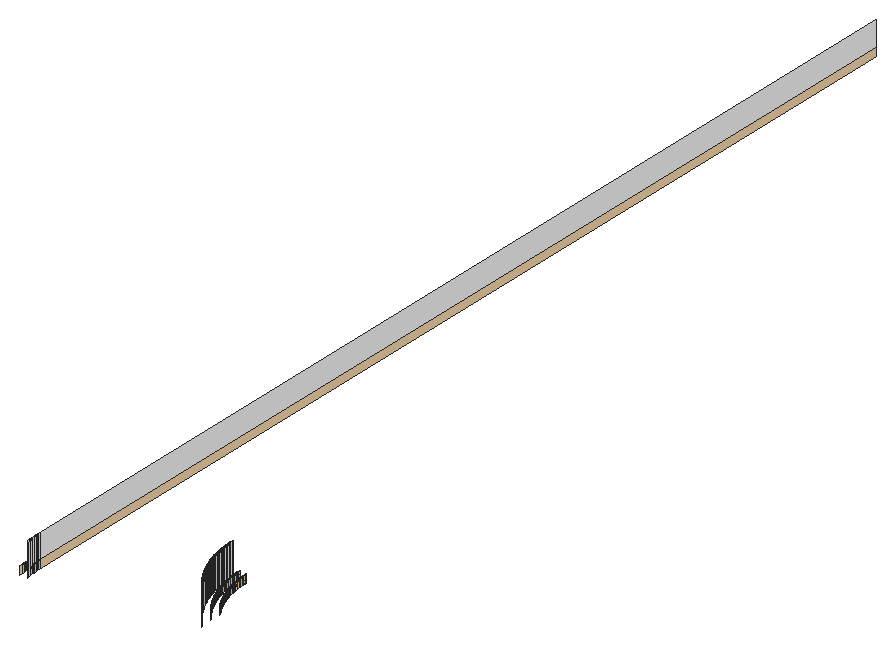
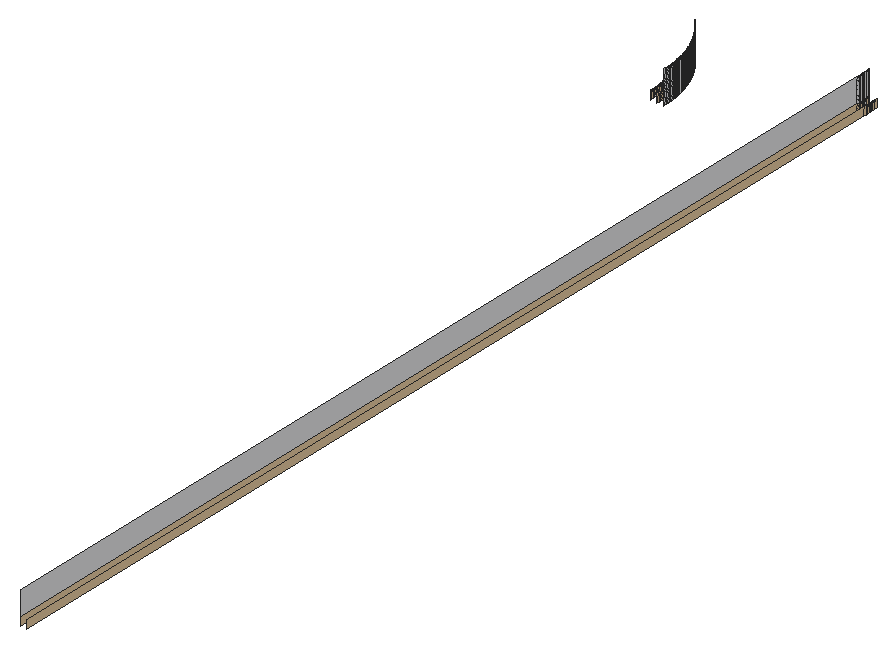
# SketchUp Ruby script. Lengths in inches.
U = 1.inch
M = Sketchup.active_model
def pt(a) = Geom::Point3d.new(a.map { |v| v * U })
def face(e, loops, mat)
  f = e.add_face(loops[0].map { |a| pt(a) })
  loops[1..].each { |l| e.add_face(l.map { |a| pt(a) }).erase! }
  f.material = f.back_material = mat if mat
  f
end
# faces: each face lists its corners as indices into pts; further lists are holes
def faces(e, pts, list, mat = nil) = list.each { |f| face(e, (f[0].is_a?(Array) ? f : [f]).map { |l| l.map { |i| pts[i] } }, mat) }
# xy, xz, yz: faces in a plane at the given z, y or x. An outline is a flat list of corners, or four numbers for a rectangle; further outlines are holes
def ring(l) = l.size == 4 ? [[l[0], l[1]], [l[2], l[1]], [l[2], l[3]], [l[0], l[3]]] : l.each_slice(2).to_a
def flat(e, list, mat, &to3) = list.each { |f| face(e, (f[0].is_a?(Array) ? f : [f]).map { |l| ring(l).map { |u, v| to3.(u, v) } }, mat) }
def xy(e, z, list, mat = nil) = flat(e, list, mat) { |x, y| [x, y, z] }
def xz(e, y, list, mat = nil) = flat(e, list, mat) { |x, z| [x, y, z] }
def yz(e, x, list, mat = nil) = flat(e, list, mat) { |y, z| [x, y, z] }
def lines(e, pts, list) = list.each { |a, b| e.add_line(pt(pts[a]), pt(pts[b])) }
# prism: a flat outline (further loops are holes) pulled along v
def prism(e, loops, v, mat = nil)
  f = face(e, loops, mat); d = Geom::Vector3d.new(v.map { |x| x * U })
  f.pushpull(f.normal.samedirection?(d) ? d.length : -d.length)
end
def box(e, o, s, mat = nil) = prism(e, [[o, [o[0] + s[0], o[1], o[2]], [o[0] + s[0], o[1] + s[1], o[2]], [o[0], o[1] + s[1], o[2]]]], [0, 0, s[2]], mat)
def at(x, y, z, deg = 0) = Geom::Transformation.translation(pt([x, y, z])) * Geom::Transformation.rotation(ORIGIN, Z_AXIS, deg.degrees)
def axes(o, x, y, z) = Geom::Transformation.new([*x, 0, *y, 0, *z, 0, *pt(o).to_a, 1])
def part(name) = M.definitions.add(name)
# library, detail: a bought-in or finely detailed component or shape, given as its bounding box
def library(name, o, s) = part(name).tap { |d| box(d.entities, o, s) }
def detail(e, o, s) = box(e.add_group.entities, o, s)
def put(e, d, t, mat = nil) = e.add_instance(d, t).tap { |i| i.material = mat if mat }
def group(e, t, mat = nil) = e.add_group.tap { |g| g.transformation = t; g.material = mat if mat }.entities
root = M.entities
M.materials.add("False Ceiling Light").color = [254, 223, 179]
M.materials.add("[Quartz Light Grey]").color = [251, 251, 252]
yz(root,22.5,[[65.53,115.32,65.76,116.49],[65.76,115.32,66,116.49],[66,115.32,216,116.49]],"False Ceiling Light")
yz(root,23.5,[[65.55,115.32,65.77,116.49],[65.77,115.32,66.01,116.49],[66.01,115.32,215.99,116.49]],"False Ceiling Light")
yz(root,23.5,[[65.55,115.32,65.77,120],[65.77,115.32,66.01,120],[66.01,115.32,215.99,120]],"[Quartz Light Grey]")
yz(root,41.5,[[77.67,115.32,77.88,120],[77.88,115.32,78.06,120]],"[Quartz Light Grey]")
yz(root,42.5,[[77.7,115.32,77.89,116.49],[77.89,115.32,78.0625,116.49]],"False Ceiling Light")
yz(root,43.5,[[77.72,115.32,77.89,116.49],[77.89,115.32,78.0625,116.49]],"False Ceiling Light")
yz(root,43.5,[[77.72,115.32,77.89,115.91],[77.89,115.32,78.0625,115.91]],"[Quartz Light Grey]")
yz(root,43.51,[[77.36,115.32,77.54,116.49]],"False Ceiling Light")
yz(root,43.51,[[77.36,115.32,77.54,115.91]],"[Quartz Light Grey]")
p = [[22.6,63.88,115.32],[22.625,63.65,115.32],[22.625,63.65,116.49],[22.6,63.88,116.49],[23.6,63.98,115.32],[23.62,63.75,115.32],
  [23.62,63.75,120],[23.6,63.98,120],[23.62,63.75,115.32],[23.6,63.98,115.32],[23.6,63.98,116.49],[23.62,63.75,116.49],
  [22.58,64.12,115.32],[22.58,64.12,116.49],[23.58,64.2,115.32],[23.58,64.2,120],[23.58,64.2,115.32],[23.58,64.2,116.49],
  [22.56,64.35,115.32],[22.56,64.35,116.49],[23.56,64.43,115.32],[23.56,64.43,120],[23.56,64.43,115.32],[23.56,64.43,116.49],
  [22.54,64.59,115.32],[22.54,64.59,116.49],[23.54,64.65,115.32],[23.54,64.65,120],[23.54,64.65,115.32],[23.54,64.65,116.49],
  [22.53,64.82,115.32],[22.53,64.82,116.49],[23.53,64.875,115.32],[23.53,64.875,120],[23.53,64.875,115.32],[23.53,64.875,116.49],
  [22.52,65.06,115.32],[22.52,65.06,116.49],[23.52,65.1,115.32],[23.52,65.1,120],[23.52,65.1,115.32],[23.52,65.1,116.49],
  [22.51,65.29,115.32],[22.51,65.29,116.49],[23.51,65.32,115.32],[23.51,65.32,120],[23.51,65.32,115.32],[23.51,65.32,116.49],
  [22.5,65.53,115.32],[22.5,65.53,116.49],[23.5,65.55,115.32],[23.5,65.55,120],[23.5,65.55,115.32],[23.5,65.55,116.49],
  [45.87,67.21,115.32],[45.73,67.36,115.32],[45.73,67.36,120],[45.87,67.21,120],[45.59,67.51,115.32],[45.59,67.51,120],
  [45.45,67.66,115.32],[45.45,67.66,120],[45.32,67.8125,115.32],[45.32,67.8125,120],[45.18,67.97,115.32],[45.18,67.97,120],
  [45.05,68.125,115.32],[45.05,68.125,120],[44.93,68.28,115.32],[44.93,68.28,120],[44.8,68.44,115.32],[44.8,68.44,120],
  [44.67,68.6,115.32],[44.67,68.6,120],[44.55,68.76,115.32],[44.55,68.76,120],[44.43,68.93,115.32],[44.43,68.93,120],
  [45.7,68.91,115.32],[45.82,68.76,115.32],[45.82,68.76,116.49],[45.7,68.91,116.49],[44.3125,69.09,115.32],[44.3125,69.09,120],
  [45.59,69.06,115.32],[45.59,69.06,116.49],[44.2,69.26,115.32],[44.2,69.26,120],[45.47,69.21,115.32],[45.47,69.21,116.49],
  [45.35,69.36,115.32],[45.35,69.36,116.49],[44.08,69.43,115.32],[44.08,69.43,120],[43.97,69.6,115.32],[43.97,69.6,120],
  [45.24,69.51,115.32],[45.24,69.51,116.49],[45.13,69.67,115.32],[45.13,69.67,116.49],[43.86,69.77,115.32],[43.86,69.77,120],
  [45.02,69.83,115.32],[45.02,69.83,116.49],[43.76,69.95,115.32],[43.76,69.95,120],[44.92,69.98,115.32],[44.92,69.98,116.49],
  [43.65,70.12,115.32],[43.65,70.12,120],[44.8125,70.14,115.32],[44.8125,70.14,116.49],[43.55,70.3,115.32],[43.55,70.3,120],
  [44.71,70.3,115.32],[44.71,70.3,116.49],[43.45,70.47,115.32],[43.45,70.47,120],[44.61,70.47,115.32],[44.61,70.47,116.49],
  [43.35,70.65,115.32],[43.35,70.65,120],[44.51,70.63,115.32],[44.51,70.63,116.49],[45.75,70.54,115.32],[45.65,70.68,115.32],
  [45.65,70.68,116.49],[45.75,70.54,116.49],[45.65,70.68,115.32],[45.75,70.54,115.32],[45.75,70.54,115.91],[45.65,70.68,115.91],
  [44.42,70.79,115.32],[44.42,70.79,116.49],[43.26,70.83,115.32],[43.26,70.83,120],[45.56,70.83,115.32],[45.56,70.83,116.49],
  [45.56,70.83,115.32],[45.56,70.83,115.91],[43.16,71.01,115.32],[43.16,71.01,120],[44.32,70.96,115.32],[44.32,70.96,116.49],
  [45.47,70.99,115.32],[45.47,70.99,116.49],[45.47,70.99,115.32],[45.47,70.99,115.91],[43.07,71.2,115.32],[43.07,71.2,120],
  [44.23,71.125,115.32],[44.23,71.125,116.49],[45.375,71.14,115.32],[45.375,71.14,116.49],[45.375,71.14,115.32],[45.375,71.14,115.91],
  [44.14,71.3,115.32],[44.14,71.3,116.49],[45.29,71.29,115.32],[45.29,71.29,116.49],[45.29,71.29,115.32],[45.29,71.29,115.91],
  [42.98,71.38,115.32],[42.98,71.38,120],[44.06,71.46,115.32],[44.06,71.46,116.49],[45.2,71.45,115.32],[45.2,71.45,116.49],
  [45.2,71.45,115.32],[45.2,71.45,115.91],[42.9,71.5625,115.32],[42.9,71.5625,120],[45.11,71.6,115.32],[45.11,71.6,116.49],
  [45.11,71.6,115.32],[45.11,71.6,115.91],[43.97,71.64,115.32],[43.97,71.64,116.49],[42.82,71.75,115.32],[42.82,71.75,120],
  [43.89,71.81,115.32],[43.89,71.81,116.49],[45.03,71.76,115.32],[45.03,71.76,116.49],[45.03,71.76,115.32],[45.03,71.76,115.91],
  [42.73,71.9375,115.32],[42.73,71.9375,120],[43.81,71.98,115.32],[43.81,71.98,116.49],[44.95,71.92,115.32],[44.95,71.92,116.49],
  [44.95,71.92,115.32],[44.95,71.92,115.91],[42.66,72.125,115.32],[42.66,72.125,120],[44.87,72.07,115.32],[44.87,72.07,116.49],
  [44.87,72.07,115.32],[44.87,72.07,115.91],[43.73,72.15,115.32],[43.73,72.15,116.49],[42.58,72.3125,115.32],[42.58,72.3125,120],
  [44.79,72.23,115.32],[44.79,72.23,116.49],[44.79,72.23,115.32],[44.79,72.23,115.91],[43.66,72.33,115.32],[43.66,72.33,116.49],
  [44.72,72.39,115.32],[44.72,72.39,116.49],[44.72,72.39,115.32],[44.72,72.39,115.91],[42.51,72.5,115.32],[42.51,72.5,120],
  [43.58,72.5,115.32],[43.58,72.5,116.49],[44.65,72.56,115.32],[44.65,72.56,116.49],[44.65,72.56,115.32],[44.65,72.56,115.91],
  [42.4375,72.69,115.32],[42.4375,72.69,120],[43.51,72.68,115.32],[43.51,72.68,116.49],[44.58,72.72,115.32],[44.58,72.72,116.49],
  [44.58,72.72,115.32],[44.58,72.72,115.91],[42.37,72.89,115.32],[42.37,72.89,120],[43.44,72.86,115.32],[43.44,72.86,116.49],
  [44.51,72.88,115.32],[44.51,72.88,116.49],[44.51,72.88,115.32],[44.51,72.88,115.91],[42.3,73.08,115.32],[42.3,73.08,120],
  [43.375,73.04,115.32],[43.375,73.04,116.49],[44.44,73.05,115.32],[44.44,73.05,116.49],[44.44,73.05,115.32],[44.44,73.05,115.91],
  [43.3125,73.22,115.32],[43.3125,73.22,116.49],[44.38,73.21,115.32],[44.38,73.21,116.49],[44.38,73.21,115.32],[44.38,73.21,115.91],
  [42.24,73.27,115.32],[42.24,73.27,120],[43.25,73.4,115.32],[43.25,73.4,116.49],[44.32,73.38,115.32],[44.32,73.38,116.49],
  [44.32,73.38,115.32],[44.32,73.38,115.91],[42.18,73.47,115.32],[42.18,73.47,120],[43.19,73.58,115.32],[43.19,73.58,116.49],
  [44.26,73.55,115.32],[44.26,73.55,116.49],[44.26,73.55,115.32],[44.26,73.55,115.91],[42.12,73.66,115.32],[42.12,73.66,120],
  [44.2,73.71,115.32],[44.2,73.71,116.49],[44.2,73.71,115.32],[44.2,73.71,115.91],[43.13,73.76,115.32],[43.13,73.76,116.49],
  [42.0625,73.86,115.32],[42.0625,73.86,120],[44.14,73.88,115.32],[44.14,73.88,116.49],[44.14,73.88,115.32],[44.14,73.88,115.91],
  [43.08,73.94,115.32],[43.08,73.94,116.49],[42.01,74.05,115.32],[42.01,74.05,120],[43.03,74.125,115.32],[43.03,74.125,116.49],
  [44.09,74.05,115.32],[44.09,74.05,116.49],[44.09,74.05,115.32],[44.09,74.05,115.91],[41.96,74.25,115.32],[41.96,74.25,120],
  [42.98,74.31,115.32],[42.98,74.31,116.49],[44.04,74.22,115.32],[44.04,74.22,116.49],[44.04,74.22,115.32],[44.04,74.22,115.91],
  [43.99,74.39,115.32],[43.99,74.39,116.49],[43.99,74.39,115.32],[43.99,74.39,115.91],[41.91,74.45,115.32],[41.91,74.45,120],
  [42.93,74.49,115.32],[42.93,74.49,116.49],[41.87,74.65,115.32],[41.87,74.65,120],[43.94,74.5625,115.32],[43.94,74.5625,116.49],
  [43.94,74.5625,115.32],[43.94,74.5625,115.91],[42.89,74.68,115.32],[42.89,74.68,116.49],[41.82,74.85,115.32],[41.82,74.85,120],
  [43.9,74.73,115.32],[43.9,74.73,116.49],[43.9,74.73,115.32],[43.9,74.73,115.91],[42.84,74.86,115.32],[42.84,74.86,116.49],
  [43.86,74.91,115.32],[43.86,74.91,116.49],[43.86,74.91,115.32],[43.86,74.91,115.91],[41.78,75.05,115.32],[41.78,75.05,120],
  [42.8,75.05,115.32],[42.8,75.05,116.49],[43.82,75.08,115.32],[43.82,75.08,116.49],[43.82,75.08,115.32],[43.82,75.08,115.91],
  [41.75,75.25,115.32],[41.75,75.25,120],[42.77,75.24,115.32],[42.77,75.24,116.49],[43.78,75.25,115.32],[43.78,75.25,116.49],
  [43.78,75.25,115.32],[43.78,75.25,115.91],[41.71,75.45,115.32],[41.71,75.45,120],[42.73,75.42,115.32],[42.73,75.42,116.49],
  [43.75,75.43,115.32],[43.75,75.43,116.49],[43.75,75.43,115.32],[43.75,75.43,115.91],[41.68,75.65,115.32],[41.68,75.65,120],
  [42.7,75.61,115.32],[42.7,75.61,116.49],[43.71,75.6,115.32],[43.71,75.6,116.49],[43.71,75.6,115.32],[43.71,75.6,115.91],
  [41.65,75.85,115.32],[41.65,75.85,120],[42.67,75.8,115.32],[42.67,75.8,116.49],[43.68,75.78,115.32],[43.68,75.78,116.49],
  [43.68,75.78,115.32],[43.68,75.78,115.91],[41.62,76.05,115.32],[41.62,76.05,120],[42.64,75.99,115.32],[42.64,75.99,116.49],
  [43.66,75.95,115.32],[43.66,75.95,116.49],[43.66,75.95,115.32],[43.66,75.95,115.91],[42.61,76.18,115.32],[42.61,76.18,116.49],
  [43.63,76.125,115.32],[43.63,76.125,116.49],[43.63,76.125,115.32],[43.63,76.125,115.91],[41.6,76.25,115.32],[41.6,76.25,120],
  [43.61,76.3,115.32],[43.61,76.3,116.49],[43.61,76.3,115.32],[43.61,76.3,115.91],[42.59,76.37,115.32],[42.59,76.37,116.49],
  [41.58,76.46,115.32],[41.58,76.46,120],[43.59,76.48,115.32],[43.59,76.48,116.49],[43.59,76.48,115.32],[43.59,76.48,115.91],
  [42.57,76.55,115.32],[42.57,76.55,116.49],[41.56,76.66,115.32],[41.56,76.66,120],[43.57,76.65,115.32],[43.57,76.65,116.49],
  [43.57,76.65,115.32],[43.57,76.65,115.91],[42.55,76.74,115.32],[42.55,76.74,116.49],[41.54,76.86,115.32],[41.54,76.86,120],
  [42.54,76.93,115.32],[42.54,76.93,116.49],[43.55,76.83,115.32],[43.55,76.83,116.49],[43.55,76.83,115.32],[43.55,76.83,115.91],
  [43.54,77.01,115.32],[43.54,77.01,116.49],[43.54,77.01,115.32],[43.54,77.01,115.91],[41.53,77.0625,115.32],[41.53,77.0625,120],
  [42.53,77.125,115.32],[42.53,77.125,116.49],[43.52,77.18,115.32],[43.52,77.18,116.49],[43.52,77.18,115.32],[43.52,77.18,115.91],
  [41.52,77.27,115.32],[41.52,77.27,120],[42.52,77.3125,115.32],[42.52,77.3125,116.49],[43.51,77.36,115.32],[43.51,77.36,116.49],
  [43.51,77.36,115.32],[43.51,77.36,115.91],[41.51,77.47,115.32],[41.51,77.47,120],[42.51,77.5,115.32],[42.51,77.5,116.49],
  [41.5,77.67,115.32],[41.5,77.67,120],[42.5,77.7,115.32],[42.5,77.7,116.49],[43.51,77.54,115.32],[43.5,77.72,115.32],
  [43.5,77.72,116.49],[43.51,77.54,116.49],[43.5,77.72,115.32],[43.51,77.54,115.32],[43.51,77.54,115.91],[43.5,77.72,115.91],
  [45.0625,66,120],[45,66,120]]
faces(root,p,[[0,1,2,3],[8,9,10,11],[12,0,3,13],[9,16,17,10],[18,12,13,19],[16,22,23,17],[24,18,19,25],[22,28,29,23],
  [30,24,25,31],[28,34,35,29],[36,30,31,37],[34,40,41,35],[42,36,37,43],[40,46,47,41],[48,42,43,49],[46,52,53,47],
  [78,79,80,81],[84,78,81,85],[88,84,85,89],[90,88,89,91],[96,90,91,97],[98,96,97,99],[102,98,99,103],[106,102,103,107],
  [110,106,107,111],[114,110,111,115],[118,114,115,119],[122,118,119,123],[124,125,126,127],[132,122,123,133],[125,136,137,126],[142,132,133,143],
  [136,144,145,137],[150,142,143,151],[144,152,153,145],[156,150,151,157],[152,158,159,153],[164,156,157,165],[158,166,167,159],[166,172,173,167],
  [176,164,165,177],[180,176,177,181],[172,182,183,173],[188,180,181,189],[182,190,191,183],[190,196,197,191],[200,188,189,201],[196,204,205,197],
  [208,200,201,209],[204,210,211,205],[216,208,209,217],[210,218,219,211],[224,216,217,225],[218,226,227,219],[232,224,225,233],[226,234,235,227],
  [240,232,233,241],[234,242,243,235],[246,240,241,247],[242,248,249,243],[254,246,247,255],[248,256,257,249],[262,254,255,263],[256,264,265,257],
  [264,270,271,265],[274,262,263,275],[270,278,279,271],[282,274,275,283],[286,282,283,287],[278,288,289,279],[294,286,287,295],[288,296,297,289],
  [296,300,301,297],[306,294,295,307],[300,310,311,301],[314,306,307,315],[310,318,319,311],[322,314,315,323],[318,324,325,319],[330,322,323,331],
  [324,332,333,325],[338,330,331,339],[332,340,341,333],[346,338,339,347],[340,348,349,341],[354,346,347,355],[348,356,357,349],[362,354,355,363],
  [356,364,365,357],[370,362,363,371],[364,372,373,365],[376,370,371,377],[372,378,379,373],[378,384,385,379],[388,376,377,389],[384,392,393,385],
  [396,388,389,397],[392,400,401,393],[404,396,397,405],[408,404,405,409],[400,410,411,401],[410,414,415,411],[420,408,409,421],[414,422,423,415],
  [428,420,421,429],[422,430,431,423],[436,428,429,437],[440,436,437,441],[442,443,444,445]],"False Ceiling Light")
faces(root,p,[[4,5,6,7],[14,4,7,15],[20,14,15,21],[26,20,21,27],[32,26,27,33],[38,32,33,39],[44,38,39,45],[50,44,45,51],
  [54,55,56,57],[55,58,59,56],[58,60,61,59],[60,62,63,61],[62,64,65,63],[64,66,67,65],[66,68,69,67],[68,70,71,69],
  [70,72,73,71],[72,74,75,73],[74,76,77,75],[76,82,83,77],[82,86,87,83],[86,92,93,87],[92,94,95,93],[94,100,101,95],
  [100,104,105,101],[104,108,109,105],[108,112,113,109],[112,116,117,113],[116,120,121,117],[128,129,130,131],[120,134,135,121],[138,128,131,139],
  [134,140,141,135],[146,138,139,147],[140,148,149,141],[154,146,147,155],[160,154,155,161],[148,162,163,149],[168,160,161,169],[162,170,171,163],
  [174,168,169,175],[170,178,179,171],[184,174,175,185],[178,186,187,179],[192,184,185,193],[186,194,195,187],[198,192,193,199],[194,202,203,195],
  [206,198,199,207],[212,206,207,213],[202,214,215,203],[220,212,213,221],[214,222,223,215],[228,220,221,229],[222,230,231,223],[236,228,229,237],
  [230,238,239,231],[244,236,237,245],[250,244,245,251],[238,252,253,239],[258,250,251,259],[252,260,261,253],[266,258,259,267],[260,268,269,261],
  [272,266,267,273],[268,276,277,269],[280,272,273,281],[276,284,285,277],[290,280,281,291],[284,292,293,285],[298,290,291,299],[302,298,299,303],
  [292,304,305,293],[304,308,309,305],[312,302,303,313],[308,316,317,309],[320,312,313,321],[326,320,321,327],[316,328,329,317],[334,326,327,335],
  [328,336,337,329],[342,334,335,343],[336,344,345,337],[350,342,343,351],[344,352,353,345],[358,350,351,359],[352,360,361,353],[366,358,359,367],
  [360,368,369,361],[374,366,367,375],[380,374,375,381],[368,382,383,369],[386,380,381,387],[382,390,391,383],[394,386,387,395],[390,398,399,391],
  [402,394,395,403],[398,406,407,399],[412,402,403,413],[416,412,413,417],[406,418,419,407],[424,416,417,425],[418,426,427,419],[432,424,425,433],
  [426,434,435,427],[434,438,439,435],[446,447,448,449]],"[Quartz Light Grey]")
lines(root,p,[[450,451]])
